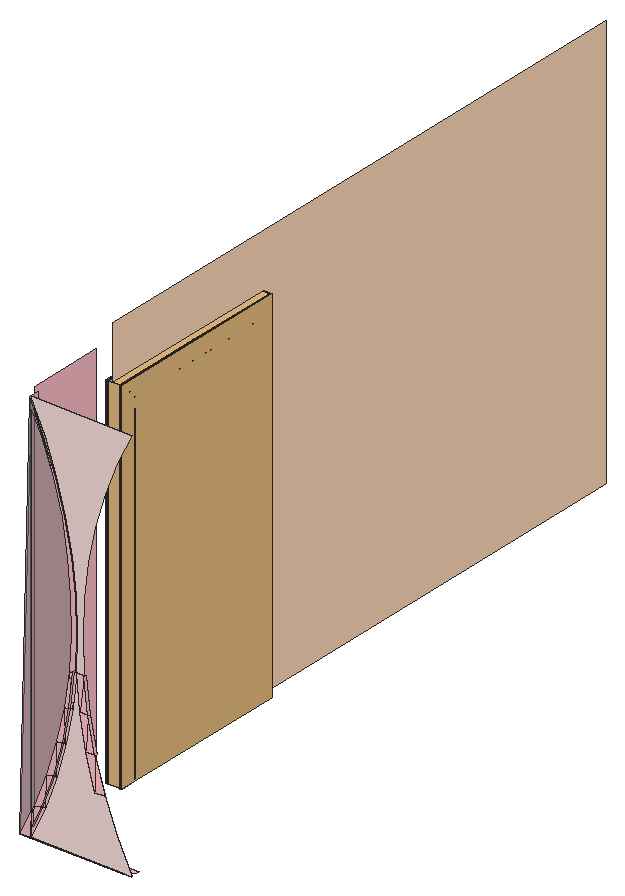
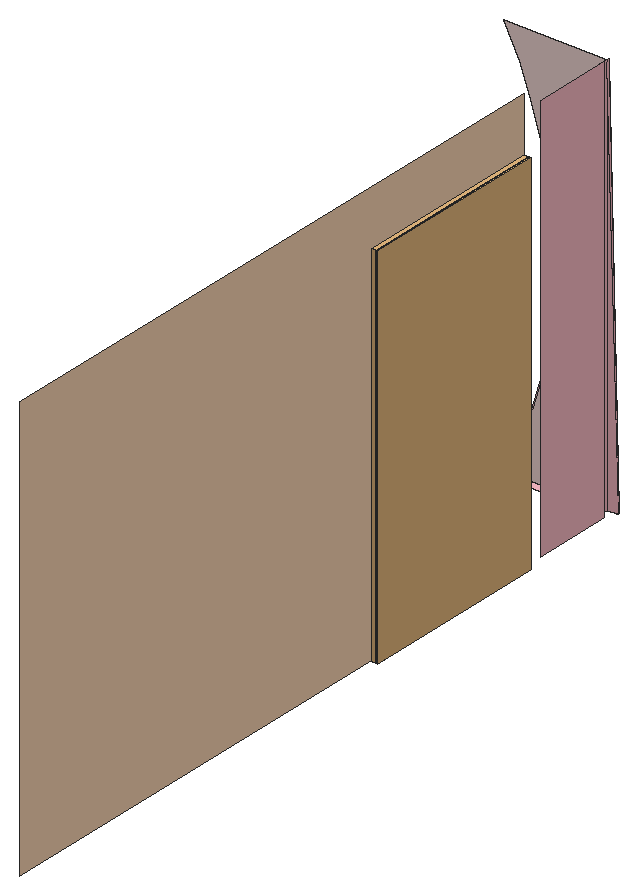
# SketchUp Ruby script. Lengths in inches.
U = 1.inch
M = Sketchup.active_model
def pt(a) = Geom::Point3d.new(a.map { |v| v * U })
def face(e, loops, mat)
  f = e.add_face(loops[0].map { |a| pt(a) })
  loops[1..].each { |l| e.add_face(l.map { |a| pt(a) }).erase! }
  f.material = f.back_material = mat if mat
  f
end
# faces: each face lists its corners as indices into pts; further lists are holes
def faces(e, pts, list, mat = nil) = list.each { |f| face(e, (f[0].is_a?(Array) ? f : [f]).map { |l| l.map { |i| pts[i] } }, mat) }
# xy, xz, yz: faces in a plane at the given z, y or x. An outline is a flat list of corners, or four numbers for a rectangle; further outlines are holes
def ring(l) = l.size == 4 ? [[l[0], l[1]], [l[2], l[1]], [l[2], l[3]], [l[0], l[3]]] : l.each_slice(2).to_a
def flat(e, list, mat, &to3) = list.each { |f| face(e, (f[0].is_a?(Array) ? f : [f]).map { |l| ring(l).map { |u, v| to3.(u, v) } }, mat) }
def xy(e, z, list, mat = nil) = flat(e, list, mat) { |x, y| [x, y, z] }
def xz(e, y, list, mat = nil) = flat(e, list, mat) { |x, z| [x, y, z] }
def yz(e, x, list, mat = nil) = flat(e, list, mat) { |y, z| [x, y, z] }
def lines(e, pts, list) = list.each { |a, b| e.add_line(pt(pts[a]), pt(pts[b])) }
# prism: a flat outline (further loops are holes) pulled along v
def prism(e, loops, v, mat = nil)
  f = face(e, loops, mat); d = Geom::Vector3d.new(v.map { |x| x * U })
  f.pushpull(f.normal.samedirection?(d) ? d.length : -d.length)
end
def box(e, o, s, mat = nil) = prism(e, [[o, [o[0] + s[0], o[1], o[2]], [o[0] + s[0], o[1] + s[1], o[2]], [o[0], o[1] + s[1], o[2]]]], [0, 0, s[2]], mat)
def at(x, y, z, deg = 0) = Geom::Transformation.translation(pt([x, y, z])) * Geom::Transformation.rotation(ORIGIN, Z_AXIS, deg.degrees)
def axes(o, x, y, z) = Geom::Transformation.new([*x, 0, *y, 0, *z, 0, *pt(o).to_a, 1])
def part(name) = M.definitions.add(name)
# library, detail: a bought-in or finely detailed component or shape, given as its bounding box
def library(name, o, s) = part(name).tap { |d| box(d.entities, o, s) }
def detail(e, o, s) = box(e.add_group.entities, o, s)
def put(e, d, t, mat = nil) = e.add_instance(d, t).tap { |i| i.material = mat if mat }
def group(e, t, mat = nil) = e.add_group.tap { |g| g.transformation = t; g.material = mat if mat }.entities
root = M.entities
M.materials.add("Material \#0").color = [86, 53, 35]
M.materials.add("Material \#1").color = [140, 140, 140]
M.materials.add("[0006_Pink]").color = [255, 192, 203]
M.materials.add("[0007_MistyRose]").color = [255, 228, 225]
M.materials.add("[0027_PeachPuff]").color = [255, 218, 185]
M.materials.add("[Translucent Glass Gray]").color = [128, 128, 128]
M.materials["[Translucent Glass Gray]"].alpha = 0.5
c1 = part("3DGeom~19_Defintion")
xy(c1.entities,0,[[-6.28,-215.79,-994.45,-208.55,-13.52,-208.55],[-994.45,-215.79,-994.45,-208.55,-6.28,-215.79],[-6.28,-215.79,-13.52,-208.55,-13.52,0],[-6.28,-215.79,-13.52,0,-6.28,0],[-13.52,0,-13.52,208.55,-6.28,215.79],
  [-13.52,0,-6.28,215.79,-6.28,0],[-994.45,208.55,-6.28,215.79,-13.52,208.55],[-994.45,208.55,-994.45,215.79,-6.28,215.79]],"Material \#0")
p = [[-13.52,-208.55,0],[-994.45,-208.55,0],[-994.45,-207.81,0.07],[-14.25,-207.81,0.07],[-13.52,-208.55,0],[-14.25,-207.81,0.07],
  [-14.25,0,0.07],[-13.52,0,0],[-13.52,208.55,0],[-14.25,207.81,0.07],[-13.52,208.55,0],[-14.25,207.81,0.07],
  [-994.45,207.81,0.07],[-994.45,208.55,0],[-994.45,-207.21,0.27],[-994.45,-207.21,0.27],[-14.86,-207.21,0.27],[-14.86,-207.21,0.27],
  [-14.86,0,0.27],[-14.86,0,0.27],[-14.86,0,0.27],[-14.86,0,0.27],[-14.86,207.21,0.27],[-14.86,207.21,0.27],
  [-994.45,207.21,0.27],[-994.45,207.21,0.27],[-14.86,-207.21,0.27],[-994.45,-207.21,0.27],[-994.45,-206.74,0.6],[-15.33,-206.74,0.6],
  [-14.86,-207.21,0.27],[-15.33,-206.74,0.6],[-15.33,0,0.6],[-14.86,0,0.27],[-14.86,207.21,0.27],[-15.33,206.74,0.6],
  [-14.86,207.21,0.27],[-15.33,206.74,0.6],[-994.45,206.74,0.6],[-994.45,207.21,0.27],[-994.45,-206.4,1.07],[-15.66,-206.4,1.07],
  [-15.66,-206.4,1.07],[-15.66,0,1.07],[-15.66,206.4,1.07],[-15.66,206.4,1.07],[-994.45,206.4,1.07],[-994.45,-206.2,1.68],
  [-15.86,-206.2,1.68],[-15.86,-206.2,1.68],[-15.86,0,1.68],[-15.86,206.2,1.68],[-15.86,206.2,1.68],[-994.45,206.2,1.68],
  [-994.45,-206.13,2.41],[-15.93,-206.13,2.41],[-15.93,-206.13,2.41],[-15.93,0,2.41],[-15.93,206.13,2.41],[-15.93,206.13,2.41],
  [-994.45,206.13,2.41],[-994.45,-206.13,71.16],[-994.45,-206.22,71.59],[-15.79,-206.28,71.53],[-15.79,-206.28,71.53],[-15.84,0,71.59],
  [-15.93,0,71.16],[-15.79,206.28,71.53],[-15.79,206.28,71.53],[-994.45,206.22,71.59],[-994.45,206.13,71.16],[-15.79,-206.28,71.53],
  [-994.45,-206.48,71.84],[-994.45,-206.9,71.93],[-15.16,-206.9,71.93],[-15.79,-206.28,71.53],[-15.79,-206.28,71.53],[-15.16,-206.9,71.93],
  [-15.16,0,71.93],[-994.45,-206.48,71.84],[-15.59,0,71.84],[-15.79,-206.28,71.53],[-15.59,0,71.84],[-15.79,206.28,71.53],
  [-15.16,206.9,71.93],[-15.59,0,71.84],[-15.79,206.28,71.53],[-994.45,206.48,71.84],[-15.79,206.28,71.53],[-15.16,206.9,71.93],
  [-994.45,206.9,71.93],[-994.45,206.48,71.84],[-15.79,206.28,71.53],[-994.45,-227.27,72.01],[5.41,-227.47,72.33],[4.78,-226.84,71.93],
  [4.78,-226.84,71.93],[5.41,-227.47,72.33],[5.21,0,72.01],[-994.45,-226.84,71.93],[-994.45,-227.27,72.01],[5.21,0,72.01],
  [4.78,0,71.93],[4.78,226.84,71.93],[5.21,0,72.01],[5.21,0,72.01],[5.41,227.47,72.33],[4.78,226.84,71.93],
  [5.41,227.47,72.33],[-994.45,227.27,72.01],[-994.45,227.27,72.01],[-994.45,226.84,71.93],[-994.45,-227.27,72.01],[-994.45,-227.53,72.27],
  [5.41,-227.47,72.33],[5.41,-227.47,72.33],[5.47,0,72.27],[5.21,0,72.01],[5.41,227.47,72.33],[5.41,227.47,72.33],
  [-994.45,227.53,72.27],[-994.45,227.27,72.01],[-994.45,-227.61,72.7],[-994.45,-227.61,74.4375],[-994.45,-227.61,74.4375],[5.55,-227.61,74.4375],
  [5.55,-227.61,74.4375],[5.55,0,74.4375],[5.55,0,72.7],[5.55,227.61,74.4375],[5.55,227.61,74.4375],[-994.45,227.61,74.4375],
  [-994.45,227.61,74.4375],[-994.45,227.61,72.7]]
faces(c1.entities,p,[[0,1,2],[2,3,0],[4,5,6],[6,7,4],[8,7,6],[6,9,8],[10,11,12],[12,13,10],
  [3,2,14],[15,16,3],[5,17,18],[19,6,5],[9,6,20],[21,22,9],[11,23,24],[25,12,11],
  [26,27,28],[28,29,26],[30,31,32],[32,33,30],[34,33,32],[32,35,34],[36,37,38],[38,39,36],
  [29,28,40],[40,41,29],[31,42,43],[43,32,31],[35,32,43],[43,44,35],[37,45,46],[46,38,37],
  [41,40,47],[47,48,41],[42,49,50],[50,43,42],[44,43,50],[50,51,44],[45,52,53],[53,46,45],
  [48,47,54],[54,55,48],[49,56,57],[57,50,49],[51,50,57],[57,58,51],[52,59,60],[60,53,52],
  [61,62,63],[64,65,66],[66,65,67],[68,69,70],[71,72,73],[73,74,75],[76,77,78],[62,79,63],
  [78,80,76],[81,82,65],[83,80,78],[78,84,83],[65,85,86],[68,87,69],[88,89,90],[90,91,92],
  [93,94,95],[96,97,98],[95,99,100],[101,102,96],[103,102,104],[105,106,103],[107,108,109],[110,111,107],
  [112,113,114],[115,116,117],[117,116,118],[119,120,121],[114,122,123],[124,125,114],[113,122,114],[115,126,127],
  [127,128,115],[115,128,116],[118,128,127],[127,129,118],[116,128,118],[119,130,131],[132,133,119],[119,133,120]],"Material \#0")
c2 = part("3DGeom~15_Defintion")
xy(c2.entities,0,[[-961.58,-251.9,-958.5,-248.8125,-961.58,-237.8],[-961.58,-251.9,28.8,-248.8125,-958.5,-248.8125],[-961.58,-251.9,36.25,-251.9,28.8,-248.8125],[36.25,-251.9,19.98,-239.99,28.8,-248.8125],[36.25,-251.9,22.16,-237.8,19.98,-239.99],
  [-958.5,-248.8125,-958.5,-237.8,-961.58,-237.8],[19.98,-239.99,22.16,-237.8,3.36,-223.37],[-958.5,-237.8,-958.5,-223.37,-961.58,-220.28],[-961.58,-237.8,-958.5,-237.8,-961.58,-220.28],[22.16,-237.8,4.64,-220.28,3.36,-223.37],
  [-958.5,-223.37,4.64,-220.28,-961.58,-220.28],[-958.5,-223.37,3.36,-223.37,4.64,-220.28],[5.29,-219.63,8.375,-218.35,5.29,0],[8.375,-218.35,8.375,0,5.29,0],[5.29,0,8.375,0,5.29,219.63],
  [8.375,0,8.375,218.35,5.29,219.63],[8.375,218.35,22.8125,237.15,5.29,219.63],[-961.58,220.28,-958.5,223.37,-961.58,237.8],[-961.58,220.28,3.36,223.37,-958.5,223.37],[-961.58,220.28,4.64,220.28,3.36,223.37],
  [4.64,220.28,19.98,239.99,3.36,223.37],[4.64,220.28,22.16,237.8,19.98,239.99],[-958.5,223.37,-958.5,237.8,-961.58,237.8],[-958.5,237.8,-958.5,248.8125,-961.58,251.9],[-961.58,237.8,-958.5,237.8,-961.58,251.9],
  [22.16,237.8,28.8,248.8125,19.98,239.99],[22.16,237.8,36.25,251.9,28.8,248.8125],[-958.5,248.8125,36.25,251.9,-961.58,251.9],[-958.5,248.8125,28.8,248.8125,36.25,251.9]],"Material \#0")
xy(c2.entities,7.48,[[-962.79,-238.36,23.37,-238.36,-962.79,-219.67],[23.37,-238.36,4.67,-219.67,-962.79,-219.67],[23.37,-238.36,23.37,0,4.67,-219.67],[4.67,-219.67,23.37,0,4.67,0],[23.37,0,23.37,238.36,4.67,219.67],
  [4.67,0,23.37,0,4.67,219.67],[-962.79,219.67,23.37,238.36,-962.79,238.36],[-962.79,219.67,4.67,219.67,23.37,238.36]],"Material \#0")
xy(c2.entities,63.5625,[[-962.79,-238.36,-962.79,-219.67,4.67,-219.67],[-962.79,-238.36,4.67,-219.67,23.37,-238.36],[23.37,-238.36,4.67,-219.67,23.37,0],[4.67,-219.67,4.67,0,23.37,0],[23.37,0,4.67,219.67,23.37,238.36],
  [4.67,0,4.67,219.67,23.37,0],[-962.79,219.67,-962.79,238.36,4.67,219.67],[4.67,219.67,-962.79,238.36,23.37,238.36]],"Material \#0")
xy(c2.entities,69.64,[[-962.79,-219.62,4.63,-219.62,-962.79,-200.32],[4.63,-219.62,-14.68,-200.32,-962.79,-200.32],[4.63,-219.62,4.63,0,-14.68,-200.32],[-14.68,-200.32,4.63,0,-14.68,0],[-14.68,0,4.63,0,-14.68,200.32],
  [4.63,0,4.63,219.62,-14.68,200.32],[-962.79,200.32,-14.68,200.32,4.63,219.62],[-962.79,200.32,4.63,219.62,-962.79,219.62]],"Material \#0")
xy(c2.entities,71.04,[[-961.58,-251.9,-958.5,-248.8125,28.8,-248.8125],[-961.58,-251.9,-961.58,-237.8,-958.5,-248.8125],[-961.58,-251.9,28.8,-248.8125,36.25,-251.9],[36.25,-251.9,19.98,-239.99,22.16,-237.8],[36.25,-251.9,28.8,-248.8125,19.98,-239.99],
  [-958.5,-248.8125,-961.58,-237.8,-958.5,-237.8],[19.98,-239.99,3.36,-223.37,22.16,-237.8],[-958.5,-237.8,-961.58,-220.28,-958.5,-223.37],[-961.58,-237.8,-961.58,-220.28,-958.5,-237.8],[22.16,-237.8,3.36,-223.37,4.64,-220.28],
  [-958.5,-223.37,-961.58,-220.28,4.64,-220.28],[-958.5,-223.37,4.64,-220.28,3.36,-223.37],[5.29,-219.63,5.29,0,8.375,-218.35],[8.375,-218.35,5.29,0,8.375,0],[5.29,0,5.29,219.63,8.375,0],
  [8.375,0,5.29,219.63,8.375,218.35],[8.375,218.35,5.29,219.63,22.8125,237.15],[-961.58,220.28,-958.5,223.37,3.36,223.37],[-961.58,220.28,-961.58,237.8,-958.5,223.37],[-961.58,220.28,3.36,223.37,4.64,220.28],
  [4.64,220.28,3.36,223.37,19.98,239.99],[4.64,220.28,19.98,239.99,22.16,237.8],[-958.5,223.37,-961.58,237.8,-958.5,237.8],[-958.5,237.8,-961.58,251.9,-958.5,248.8125],[-961.58,237.8,-961.58,251.9,-958.5,237.8],
  [22.16,237.8,19.98,239.99,28.8,248.8125],[22.16,237.8,28.8,248.8125,36.25,251.9],[-958.5,248.8125,-961.58,251.9,36.25,251.9],[-958.5,248.8125,36.25,251.9,28.8,248.8125]],"Material \#0")
xz(c2.entities,-238.36,[[-962.79,63.5625,23.37,63.5625,23.37,72.07],[-962.79,63.5625,23.37,72.07,-962.79,72.07]],"Material \#0")
xz(c2.entities,-219.67,[[-962.79,7.48,4.67,7.48,-962.79,63.5625],[4.67,7.48,4.67,63.5625,-962.79,63.5625]],"Material \#0")
xz(c2.entities,219.67,[[-962.79,7.48,-962.79,63.5625,4.67,7.48],[4.67,7.48,-962.79,63.5625,4.67,63.5625]],"Material \#0")
xz(c2.entities,238.36,[[-962.79,63.5625,-962.79,72.07,23.37,72.07],[-962.79,63.5625,23.37,72.07,23.37,63.5625]],"Material \#0")
yz(c2.entities,4.67,[[-219.67,7.48,0,7.48,-219.67,63.5625],[0,7.48,0,63.5625,-219.67,63.5625],[0,7.48,219.67,63.5625,0,63.5625],[0,7.48,219.67,7.48,219.67,63.5625]],"Material \#0")
yz(c2.entities,23.37,[[-238.36,63.5625,0,63.5625,-238.36,72.07],[0,63.5625,0,72.07,-238.36,72.07],[0,63.5625,238.36,63.5625,238.36,72.07],[0,63.5625,238.36,72.07,0,72.07]],"Material \#0")
p = [[36.9,-251.24,0],[37.21,0,-0.16],[34.125,0,-0.14],[36.9,251.24,0],[33.83,243.81,0.02],[33.83,-243.8,0.02],
  [22.8125,-237.15,0],[24.99,-234.97,-0.01],[5.375,-220.37,0],[23.37,-238.36,7.48],[4.67,-219.67,7.48],[4.67,-219.67,7.48],
  [23.37,-238.36,7.48],[23.37,-238.36,0],[4.67,-219.67,7.48],[23.37,-238.36,0],[5.375,-220.37,0],[5.375,-220.37,0],
  [23.37,-238.36,0],[5.29,-219.63,0],[8.375,-218.35,0],[-15.36,-199.64,1.62],[4.67,-219.67,7.48],[5.375,-220.37,0],
  [-13.8,-201.19,0.06],[5.375,-220.37,0],[5.375,-220.37,0],[-14.84,-200.15,0.58],[5.375,-220.37,0],[-13.8,-201.19,0.06],
  [-6.08,-208.92,0],[5.375,-220.37,0],[-13.8,-201.19,0.06],[-6.08,-208.92,0],[-13.8,-201.19,0.06],[5.375,-220.37,0],
  [-6.08,-208.92,0],[-13.8,-201.19,0.06],[-13.09,-201.91,0],[-6.08,-208.92,0],[-13.09,-201.91,0],[-13.8,-201.19,0.06],
  [-15.36,199.64,1.62],[4.67,219.67,7.48],[5.375,220.37,0],[-13.8,201.19,0.06],[5.375,220.37,0],[5.375,220.37,0],
  [4.67,219.67,7.48],[-14.84,200.15,0.58],[5.375,220.37,0],[-13.8,201.19,0.06],[-6.08,208.92,0],[-13.09,201.91,0],
  [-13.8,201.19,0.06],[-6.08,208.92,0],[-13.8,201.19,0.06],[5.375,220.37,0],[-6.08,208.92,0],[5.375,220.37,0],
  [-13.8,201.19,0.06],[-6.08,208.92,0],[-13.8,201.19,0.06],[-13.09,201.91,0],[8.375,218.35,0],[24.99,234.97,-0.01],
  [22.8125,237.15,0],[23.37,238.36,7.48],[23.37,238.36,0],[23.37,238.36,0],[5.375,220.37,0],[5.375,220.37,0],
  [23.37,238.36,7.48],[4.67,219.67,7.48],[5.375,220.37,0],[23.37,238.36,0],[23.37,238.36,7.48],[-13.8,-201.19,0.06],
  [-14.84,-200.15,0.58],[-14.38,-200.61,0.26],[-13.8,-201.19,0.06],[-13.8,-201.19,0.06],[-14.38,-200.61,0.26],[-13.8,201.19,0.06],
  [-14.84,200.15,0.58],[-13.8,201.19,0.06],[-14.38,200.61,0.26],[-14.38,200.61,0.26],[-13.8,201.19,0.06],[4.63,-219.62,69.64],
  [4.63,-219.62,69.64],[-15.42,-199.57,9.43],[-15.36,-199.64,1.62],[-15.16,-199.83,1.04],[-15.16,-199.83,1.04],[-15.16,199.83,1.04],
  [-15.36,199.64,1.62],[-15.16,199.83,1.04],[-15.42,199.57,9.43],[4.63,219.62,69.64],[4.67,219.67,7.48],[4.63,219.62,69.64],
  [4.63,-219.62,69.64],[4.67,-219.67,63.5625],[4.67,-219.67,63.5625],[4.67,-219.67,7.48],[-15.28,-199.71,69.25],[4.63,-219.62,69.64],
  [-15.42,-199.57,9.43],[-15.28,-199.71,69.25],[-15.42,-199.57,2.34],[-15.42,-199.57,2.34],[-15.42,199.57,2.34],[-15.42,199.57,9.43],
  [-15.28,199.71,69.25],[-15.28,199.71,69.25],[4.63,219.62,69.64],[4.63,219.62,69.64],[4.67,219.67,63.5625],[4.67,219.67,63.5625],
  [-15.42,199.57,2.34],[4.67,-219.67,63.5625],[4.63,-219.62,69.64],[4.67,219.67,7.48],[4.67,219.67,63.5625],[4.63,219.62,69.64],
  [4.63,-219.62,69.64],[-15.28,-199.71,69.25],[-15.28,-199.71,69.25],[-15.42,-199.57,48.99],[-15.42,-199.57,48.99],[-15.28,-199.71,69.25],
  [-15.42,199.57,48.99],[-15.28,199.71,69.25],[-15.28,199.71,69.25],[-15.42,199.57,48.99],[4.63,219.62,69.64],[4.63,-219.62,69.64],
  [23.37,-238.36,72.07],[4.67,-219.67,63.5625],[4.67,-219.67,63.5625],[23.37,-238.36,63.5625],[23.37,-238.36,72.07],[4.67,-219.67,63.5625],
  [5.24,-220.23,70.03],[23.37,-238.36,72.07],[23.37,-238.36,63.5625],[4.67,-219.67,63.5625],[4.67,-219.67,63.5625],[4.63,-219.62,69.64],
  [4.63,219.62,69.64],[23.37,238.36,72.07],[4.67,219.67,63.5625],[4.67,219.67,63.5625],[5.24,220.23,70.03],[4.63,219.62,69.64],
  [23.37,238.36,63.5625],[4.67,219.67,63.5625],[4.67,219.67,63.5625],[23.37,238.36,63.5625],[23.37,238.36,72.07],[4.67,219.67,63.5625],
  [23.37,238.36,72.07],[4.63,-219.62,69.64],[-14.68,-200.32,69.64],[-15.28,-199.71,69.25],[-15.28,-199.71,69.25],[-14.68,-200.32,69.64],
  [4.63,-219.62,69.64],[-15.28,199.71,69.25],[-14.68,200.32,69.64],[4.63,219.62,69.64],[4.63,219.62,69.64],[-14.68,200.32,69.64],
  [4.63,-219.62,69.64],[5.24,-220.23,70.03],[23.37,-238.36,72.07],[4.63,219.62,69.64],[5.24,220.23,70.03],[5.375,-220.37,72.07],
  [5.375,-220.37,72.07],[23.37,-238.36,72.07],[5.375,220.37,72.07],[23.37,238.36,72.07],[5.375,220.37,72.07],[33.83,-243.8,71.03],
  [36.9,-251.24,71.04],[22.8125,-237.15,71.04],[34.125,0,71.19],[37.21,0,71.2],[24.99,-234.97,71.05],[5.29,-219.63,71.04],
  [8.375,-218.35,71.04],[33.83,243.81,71.03],[36.9,251.24,71.04],[22.8125,237.15,71.04],[24.99,234.97,71.05],[8.375,218.35,71.04]]
faces(c2.entities,p,[[0,1,2],[1,3,4],[4,2,1],[2,5,0],[6,0,5],[5,7,6],[8,9,10],[11,12,13],
  [14,15,16],[17,18,9],[19,6,7],[7,20,19],[21,22,23],[24,21,25],[26,10,27],[28,27,29],
  [30,31,32],[33,34,35],[36,37,38],[39,40,41],[42,43,44],[45,42,46],[47,48,49],[50,49,51],
  [52,53,54],[55,56,57],[58,59,60],[61,62,63],[64,65,66],[43,67,68],[43,69,70],[71,72,73],
  [74,75,76],[3,66,65],[65,4,3],[77,78,21],[27,79,80],[81,82,78],[83,84,42],[85,86,84],
  [49,87,88],[10,89,27],[90,91,27],[92,93,27],[91,92,27],[78,94,21],[84,95,42],[96,97,49],
  [98,96,49],[99,98,49],[100,101,49],[21,102,103],[21,104,105],[21,106,107],[21,108,109],[91,110,92],
  [21,111,108],[42,112,113],[42,113,114],[42,115,116],[42,117,118],[42,119,43],[98,120,96],[10,121,122],
  [123,124,125],[126,127,91],[128,129,91],[108,130,131],[113,132,133],[134,135,98],[136,134,98],[137,138,139],
  [140,141,142],[143,142,144],[145,146,147],[148,144,149],[150,151,152],[153,154,155],[151,156,157],[158,159,160],
  [161,162,154],[163,164,165],[166,167,168],[169,170,171],[172,173,134],[174,175,176],[177,178,151],[142,179,144],
  [175,180,181],[178,182,151],[183,184,154],[185,186,187],[186,185,188],[188,189,186],[187,190,185],[190,187,191],
  [191,192,190],[189,188,193],[193,194,189],[195,196,197],[196,195,194],[194,193,196]],"Material \#0")
c3 = part("3DGeom~22_Defintion")
xz(c3.entities,-210.625,[[-1016.13,2.47,-1016.13,9.96,-16.28,2.47],[-16.28,2.47,-1016.13,9.96,-16.28,9.96],[-1016.13,9.96,-1016.13,51.7,-16.28,51.7],[-1016.13,9.96,-16.28,51.7,-16.28,9.96],[-1016.13,51.7,-1016.13,72.71,-16.28,51.7]],"Material \#0")
xz(c3.entities,210.625,[[-1016.13,2.47,-16.28,2.47,-1016.13,9.96],[-16.28,2.47,-16.28,9.96,-1016.13,9.96],[-1016.13,9.96,-16.28,51.7,-1016.13,51.7],[-1016.13,9.96,-16.28,9.96,-16.28,51.7],[-1016.13,51.7,-16.28,51.7,-1016.13,72.71]],"Material \#0")
yz(c3.entities,-16.28,[[-210.625,2.47,-210.625,9.96,0,9.96],[-210.625,2.47,0,9.96,0,2.47],[0,2.47,0,9.96,210.625,2.47],[210.625,2.47,0,9.96,210.625,9.96],[-210.625,9.96,-210.625,51.7,0,51.7],
  [-210.625,9.96,0,51.7,0,9.96],[0,9.96,0,51.7,210.625,9.96],[210.625,9.96,0,51.7,210.625,51.7],[-210.625,51.7,0,72.71,0,51.7],[0,51.7,0,72.71,210.625,51.7]],"Material \#0")
p = [[-1016.13,-210.625,72.71],[-16.13,-210.77,73.09],[-16.28,-210.625,51.7],[-16.28,-210.625,51.7],[-16.13,-210.77,73.09],[-16.28,0,72.71],
  [-16.13,210.77,73.09],[-16.28,210.625,51.7],[-16.28,210.625,51.7],[-16.13,210.77,73.09],[-1016.13,210.625,72.71]]
faces(c3.entities,p,[[0,1,2],[3,4,5],[5,6,7],[8,9,10]],"Material \#0")
c4 = library("3DGeom~16_Defintion",[-962.62,-252.34,-11.22],[1000,504.68,93.46])
c5 = part("3DGeom~17_Defintion")
yz(c5.entities,-1908.8,[[-436.03,-21.87,-436.73,-21.5,-435.91,-21.83],[436.03,-21.87,435.91,-21.83,436.73,-21.5],[-435.91,-21.83,-436.73,-21.5,-436.15,-21.125],[-435.91,-21.83,-436.15,-21.125,-435.87,-21.72],[435.91,-21.83,435.87,-21.72,436.15,-21.125],
  [435.91,-21.83,436.15,-21.125,436.73,-21.5],[-436.73,-21.5,-484.73,-21.37,-436.15,-1.11],[-471.46,-21.5,-484.73,-21.37,-436.73,-21.5],[-477.2,-21.5,-484.73,-21.37,-471.46,-21.5],[-481.82,-21.5,-484.73,-21.37,-477.2,-21.5],
  [-436.73,-21.5,-436.15,-1.11,-436.15,-21.125],[436.73,-21.5,436.15,-21.125,471.46,-21.5],[471.46,-21.5,436.15,-21.125,477.2,-21.5],[477.2,-21.5,436.15,-21.125,499.98,-0.85],[477.2,-21.5,499.98,-0.85,481.82,-21.5],
  [481.82,-21.5,487.35,-21,484.73,-21.37],[481.82,-21.5,491.8,-19.52,487.35,-21],[481.82,-21.5,497.64,-13.67,491.8,-19.52],[481.82,-21.5,499.98,-0.85,497.64,-13.67],[-484.73,-21.37,-498.5,-11.58,-499.84,-0.37],
  [-484.73,-21.37,-499.84,-0.37,-499.4,-0.5],[-484.73,-21.37,-499.4,-0.5,-436.15,-1.11],[-484.73,-21.37,-493.63,-18.42,-498.5,-11.58],[-484.73,-21.37,-489.71,-20.375,-493.63,-18.42],[-484.73,-21.37,-487.35,-21,-489.71,-20.375],
  [436.15,-21.125,436.15,-1.11,436.73,-0.74],[436.15,-21.125,436.73,-0.74,499.98,-0.85],[487.35,-21,491.8,-19.52,489.71,-20.375],[-489.71,-20.375,-491.8,-19.52,-493.63,-18.42],[491.8,-19.52,495.21,-17.08,493.63,-18.42],
  [491.8,-19.52,497.64,-13.67,495.21,-17.08],[-493.63,-18.42,-496.54,-15.5,-498.5,-11.58],[-493.63,-18.42,-495.21,-17.08,-496.54,-15.5],[495.21,-17.08,497.64,-13.67,496.54,-15.5],[-496.54,-15.5,-497.64,-13.67,-498.5,-11.58],
  [497.64,-13.67,499.125,-9.22,498.5,-11.58],[497.64,-13.67,499.625,-3.69,499.125,-9.22],[497.64,-13.67,499.98,-0.85,499.625,-3.69],[-498.5,-11.58,-499.625,-3.69,-499.84,-0.37],[-498.5,-11.58,-499.5,-6.6,-499.625,-3.69],
  [-498.5,-11.58,-499.125,-9.22,-499.5,-6.6],[499.125,-9.22,499.625,-3.69,499.5,-6.6],[-499.625,-3.69,-499.98,-0.85,-500,-0.52],[-499.625,-3.69,-500,-0.52,-499.84,-0.37],[-436.15,-1.11,-499.4,-0.5,-471.46,-0.74],
  [-436.15,-1.11,-471.46,-0.74,-436.73,-0.74],[-436.15,-1.11,-436.73,-0.74,-435.91,-0.41],[-436.15,-1.11,-435.91,-0.41,-435.87,-0.52],[436.15,-1.11,435.87,-0.52,435.91,-0.41],[436.15,-1.11,435.91,-0.41,436.73,-0.74],
  [499.98,-0.85,436.73,-0.74,471.46,-0.74],[499.98,-0.85,471.46,-0.74,499.4,-0.5],[499.98,-0.85,499.4,-0.5,499.96,-0.41],[499.98,-0.85,499.96,-0.41,500,-0.52],[-436.73,-0.74,-436.03,-0.37,-435.91,-0.41],
  [436.73,-0.74,435.91,-0.41,436.03,-0.37],[-500,-0.52,-499.96,-0.41,-499.84,-0.37],[499.4,-0.5,499.84,-0.37,499.96,-0.41],[-499.84,141.21,-499.96,141.25,-499.4,141.35],[-436.03,141.21,-436.73,141.59,-435.91,141.25],
  [436.03,141.21,435.91,141.25,436.73,141.59],[499.84,141.21,484.73,162.21,498.5,152.42],[499.84,141.21,499.4,141.35,484.73,162.21],[499.84,141.21,498.5,152.42,499.625,144.53],[499.84,141.21,499.625,144.53,500,141.37],
  [499.84,141.21,500,141.37,499.96,141.25],[-499.96,141.25,-500,141.37,-499.98,141.69],[-499.96,141.25,-499.98,141.69,-499.4,141.35],[-435.91,141.25,-436.73,141.59,-436.15,141.96],[-435.91,141.25,-436.15,141.96,-435.87,141.37],
  [435.91,141.25,435.87,141.37,436.15,141.96],[435.91,141.25,436.15,141.96,436.73,141.59],[-499.4,141.35,-499.98,141.69,-471.46,141.59],[499.4,141.35,436.15,141.96,484.73,162.21],[499.4,141.35,471.46,141.59,436.15,141.96],
  [500,141.37,499.625,144.53,499.98,141.69],[-436.73,141.59,-499.98,141.69,-436.15,161.97],[-471.46,141.59,-499.98,141.69,-436.73,141.59],[-436.73,141.59,-436.15,161.97,-436.15,141.96],[436.73,141.59,436.15,141.96,471.46,141.59],
  [-499.98,141.69,-477.2,162.34,-436.15,161.97],[-499.98,141.69,-481.82,162.34,-477.2,162.34],[-499.98,141.69,-497.64,154.51,-481.82,162.34],[-499.98,141.69,-499.625,144.53,-497.64,154.51],[436.15,141.96,436.15,161.97,436.73,162.34],
  [436.15,141.96,436.73,162.34,484.73,162.21],[-499.625,144.53,-499.125,150.07,-497.64,154.51],[-499.625,144.53,-499.5,147.44,-499.125,150.07],[499.625,144.53,498.5,152.42,499.5,147.44],[499.5,147.44,498.5,152.42,499.125,150.07],
  [-499.125,150.07,-498.5,152.42,-497.64,154.51],[498.5,152.42,484.73,162.21,493.63,159.26],[498.5,152.42,493.63,159.26,496.54,156.34],[498.5,152.42,496.54,156.34,497.64,154.51],[-497.64,154.51,-491.8,160.36,-481.82,162.34],
  [-497.64,154.51,-495.21,157.92,-491.8,160.36],[-497.64,154.51,-496.54,156.34,-495.21,157.92],[496.54,156.34,493.63,159.26,495.21,157.92],[-495.21,157.92,-493.63,159.26,-491.8,160.36],[493.63,159.26,484.73,162.21,489.71,161.22],
  [493.63,159.26,489.71,161.22,491.8,160.36],[-491.8,160.36,-487.35,161.84,-481.82,162.34],[-491.8,160.36,-489.71,161.22,-487.35,161.84],[489.71,161.22,484.73,162.21,487.35,161.84],[-487.35,161.84,-484.73,162.21,-481.82,162.34],
  [-436.15,161.97,-477.2,162.34,-471.46,162.34],[-436.15,161.97,-471.46,162.34,-436.73,162.34],[-436.15,161.97,-436.73,162.34,-435.91,162.68],[-436.15,161.97,-435.91,162.68,-435.87,162.56],[436.15,161.97,435.87,162.56,435.91,162.68],
  [436.15,161.97,435.91,162.68,436.73,162.34],[484.73,162.21,436.73,162.34,471.46,162.34],[484.73,162.21,471.46,162.34,477.2,162.34],[484.73,162.21,477.2,162.34,481.82,162.34],[-436.73,162.34,-436.03,162.72,-435.91,162.68],
  [436.73,162.34,435.91,162.68,436.03,162.72]],"Material \#0")
c6 = part("3DGeom~18_Defintion")
xz(c6.entities,-241.71,[[-976.3,0,23.7,0,23.7,7.58],[-976.3,0,23.7,7.58,-976.3,7.58]],"Material \#0")
xz(c6.entities,241.71,[[-976.3,0,-976.3,7.58,23.7,7.58],[-976.3,0,23.7,7.58,23.7,0]],"Material \#0")
yz(c6.entities,23.7,[[-241.71,0,0,0,-241.71,7.58],[0,0,0,7.58,-241.71,7.58],[0,0,241.71,0,241.71,7.58],[0,0,241.71,7.58,0,7.58]],"Material \#0")
c7 = part("3DGeom~20_Defintion")
xy(c7.entities,0,[[-976.3,-241.71,-976.3,-223.46,23.7,-241.71],[23.7,-241.71,-976.3,-223.46,5.45,-223.46],[23.7,-241.71,5.45,-223.46,5.45,0],[23.7,-241.71,5.45,0,23.7,0],[-976.3,-223.46,-976.3,-211.85,5.45,-223.46],
  [5.45,-223.46,-976.3,-211.85,-6.16,-211.85],[5.45,-223.46,-6.16,-211.85,-6.16,0],[5.45,-223.46,-6.16,0,5.45,0],[-6.16,0,-6.16,211.85,5.45,223.46],[-6.16,0,5.45,223.46,5.45,0],
  [5.45,0,23.7,241.71,23.7,0],[5.45,0,5.45,223.46,23.7,241.71],[-976.3,211.85,-976.3,223.46,5.45,223.46],[-976.3,211.85,5.45,223.46,-6.16,211.85],[-976.3,223.46,-976.3,241.71,23.7,241.71],
  [-976.3,223.46,23.7,241.71,5.45,223.46]],"Material \#0")
xy(root,0.5,[[362.67,320.52,365.5625,321.02,393.03,321.02,392.64,320.625,392.04,320.52],[365.5625,321.02,365.5625,323.46,394.9375,323.46,394.9375,322.95,393.03,321.02]],"[0006_Pink]")
xz(root,320.52,[[362.67,0.5,366.23,7.87,366.23,112.72,369.05,106.49,372.43,97.17,374.26,90.58,372.61,97.1875,369.45,106.64,365.5625,115.8125],[366.23,7.87,367.01,9.47,370.64,18.75,373.54,28.28,375.7,38.01,377.1,47.87,377.74,57.8125,377.6,67.78,376.7,77.7,375.03,87.52,374.26,90.58,372.43,97.17,369.05,106.49,366.23,112.72]],"[Translucent Glass Gray]")
xz(root,321.02,[[366.23,3.59,369.05,9.82,372.43,19.14,375.08,28.6875,376.99,38.41,378.14,48.25,378.52,58.16,378.14,68.06,376.99,77.9,375.08,87.625,372.43,97.17,369.05,106.49,366.23,112.72]],"[0006_Pink]")
xz(root,321.02,[[365.5625,0.5,394.9375,0.5,390.59,9.51,386.99,18.84,384.16,28.4375,382.13,38.23,380.91,48.16,380.5,58.16,380.91,68.15,382.13,78.08,384.16,87.875,386.99,97.47,390.59,106.8,394.9375,115.8125,365.5625,115.8125,369.67,106.74,373.07,97.375,375.73,87.78,377.65,78,378.8,68.11,379.1875,58.16,378.8,48.2,377.65,38.31,375.73,28.53,373.07,18.9375,369.67,9.57]],"[0007_MistyRose]")
yz(root,364.03,[[398.02,43.52,397.86,43.55,398.02,43.53],[398.02,43.52,398.02,43.53,398.18,43.53],[398.02,43.53,398.17,43.55,398.18,43.53],[398.18,43.53,398.17,43.55,398.33,43.57],[398.17,43.55,398.32,43.59,398.33,43.57],
  [398.33,43.57,398.32,43.59,398.46,43.64],[398.32,43.59,398.46,43.65,398.46,43.64],[398.46,43.64,398.46,43.65,398.59,43.72],[398.46,43.65,398.58,43.73,398.59,43.72],[398.59,43.72,398.58,43.73,398.69,43.83],
  [398.58,43.73,398.68,43.84,398.69,43.83],[397.96,43.75,397.91,43.77,397.92,43.78],[398.02,43.75,398.02,43.76,398.07,43.75],[398.07,43.75,398.02,43.76,398.07,43.77],[398.07,43.75,398.07,43.77,398.12,43.77],
  [397.91,43.77,397.87,43.79,397.875,43.8],[397.91,43.77,397.875,43.8,397.92,43.78],[398.07,43.77,398.11,43.78,398.12,43.77],[398.12,43.77,398.11,43.78,398.17,43.79],[398.11,43.78,398.16,43.8,398.17,43.79],
  [397.87,43.79,397.83,43.82,397.84,43.83],[397.87,43.79,397.84,43.83,397.875,43.8],[397.83,43.82,397.79,43.85,397.8,43.86],[397.83,43.82,397.8,43.86,397.84,43.83],[398.69,43.83,398.68,43.84,398.78,43.9375],
  [398.68,43.84,398.76,43.95,398.78,43.9375],[397.79,43.85,397.78,43.9,397.8,43.86],[398.24,43.85,398.23,43.86,398.27,43.89],[398.23,43.86,398.26,43.9,398.27,43.89],[398.27,43.89,398.26,43.9,398.29,43.9375],
  [398.26,43.9,398.28,43.94,398.29,43.9375],[398.29,43.9375,398.28,43.94,398.31,43.99],[398.78,43.9375,398.76,43.95,398.85,44.08],[398.28,43.94,398.29,43.99,398.31,43.99],[398.76,43.95,398.83,44.09,398.85,44.08],
  [398.29,43.99,398.3,44.03,398.3125,44.03],[398.29,43.99,398.3125,44.03,398.31,43.99],[398.3,44.03,398.29,44.08,398.31,44.09],[398.3,44.03,398.31,44.09,398.3125,44.03],[398.29,44.08,398.28,44.13,398.29,44.14],
  [398.29,44.08,398.29,44.14,398.31,44.09],[398.85,44.08,398.83,44.09,398.89,44.23],[398.83,44.09,398.875,44.23,398.89,44.23],[398.28,44.13,398.26,44.17,398.27,44.18],[398.28,44.13,398.27,44.18,398.29,44.14],
  [398.26,44.17,398.24,44.22,398.27,44.18],[397.8,44.21,397.79,44.22,397.84,44.24],[397.79,44.22,397.83,44.26,397.84,44.24],[398.875,44.23,398.89,44.39,398.9,44.39],[398.875,44.23,398.9,44.39,398.89,44.23],
  [397.84,44.24,397.83,44.26,397.875,44.27],[397.91,44.3,397.96,44.32,397.97,44.3]],"Material \#1")
yz(root,364.5625,[[323.46,0,345.9375,116.8125]],"[0006_Pink]")
yz(root,364.5625,[[406.625,0,531.9375,0,531.9375,121.1875,351.9375,121.1875,351.9375,105.53,406.625,105.53]],"[0027_PeachPuff]")
yz(root,365.5625,[[321.02,0.5,323.46,115.8125]],"[0006_Pink]")
yz(root,366.23,[[320.52,3.59,321.02,112.72]],"[0006_Pink]")
p = [[365.5625,320.52,115.8125],[365.5625,321.02,115.8125],[362.67,320.52,0.5],[365.5625,321.02,0.5],[367.01,320.52,9.47],[366.23,320.52,7.87],
  [369.67,321.02,9.57],[369.05,321.02,9.82],[366.23,321.02,3.59],[366.23,320.52,3.59],[369.05,320.52,9.82],[370.64,320.52,18.75],
  [373.07,321.02,18.9375],[372.43,321.02,19.14],[372.43,320.52,19.14],[373.54,320.52,28.28],[386.99,321.02,18.84],[384.55,320.52,19.04],
  [384.16,321.02,28.4375],[375.73,321.02,28.53],[381.97,320.52,28.71],[375.08,321.02,28.6875],[375.08,320.52,28.6875],[375.7,320.52,38.01],
  [382.13,321.02,38.23],[377.65,321.02,38.31],[384.63,321.02,28.56],[382.61,321.02,38.3125],[382.61,320.52,38.3125],[384.63,320.52,28.56],
  [376.99,321.02,38.41],[376.99,320.52,38.41],[380.18,320.52,38.55],[377.1,320.52,47.87],[380.91,321.02,48.16],[378.8,321.02,48.2],
  [381.39,321.02,48.2],[381.39,320.52,48.2],[378.14,321.02,48.25],[378.14,320.52,48.25],[379.21,320.52,48.51]]
faces(root,p,[[0,1,2],[3,2,1],[2,3,4,5],[6,4,3],[7,8,9,10],[4,6,11],[12,11,6],[13,7,10,14],
  [11,12,15],[16,17,18],[19,15,12],[20,18,17],[21,13,14,22],[15,19,23],[18,20,24],[25,23,19],
  [26,27,28,29],[30,21,22,31],[32,24,20],[23,25,33],[24,32,34],[35,33,25],[27,36,37,28],[38,30,31,39],
  [40,34,32]],"[0006_Pink]")
put(root,c1,axes([366.71,379.28,101.58],[0,0,0.10215],[0,-0.10489,0],[-0.0475,0,0]),"Material \#0")
put(root,c2,axes([366.71,379.28,101.58],[0,0,0.10551],[0,-0.10834,0],[-0.04906,0,0]),"Material \#0")
put(root,c3,axes([366.71,379.28,101.58],[0,0,0.09997],[0,-0.10265,0],[-0.04648,0,0]),"Material \#0")
put(root,c4,axes([366.71,379.28,101.58],[0,0,0.10553],[0,-0.10836,0],[-0.04907,0,0]),"Material \#0")
put(root,c5,axes([366.71,379.28,101.58],[0,0,0.05322],[0,-0.05465,0],[-0.02475,0,0]),"Material \#0")
put(root,c6,axes([366.71,379.28,101.58],[0,0,0.10405],[0,-0.10684,0],[-0.04838,0,0]),"Material \#0")
put(root,c7,axes([366.71,379.28,101.58],[0,0,0.10405],[0,-0.10684,0],[-0.04838,0,0]),"Material \#0")
